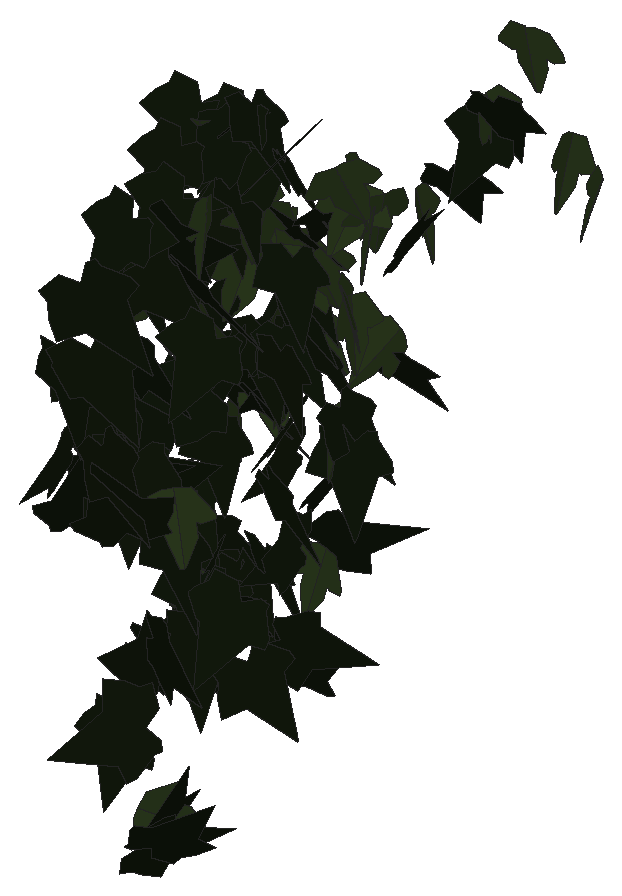
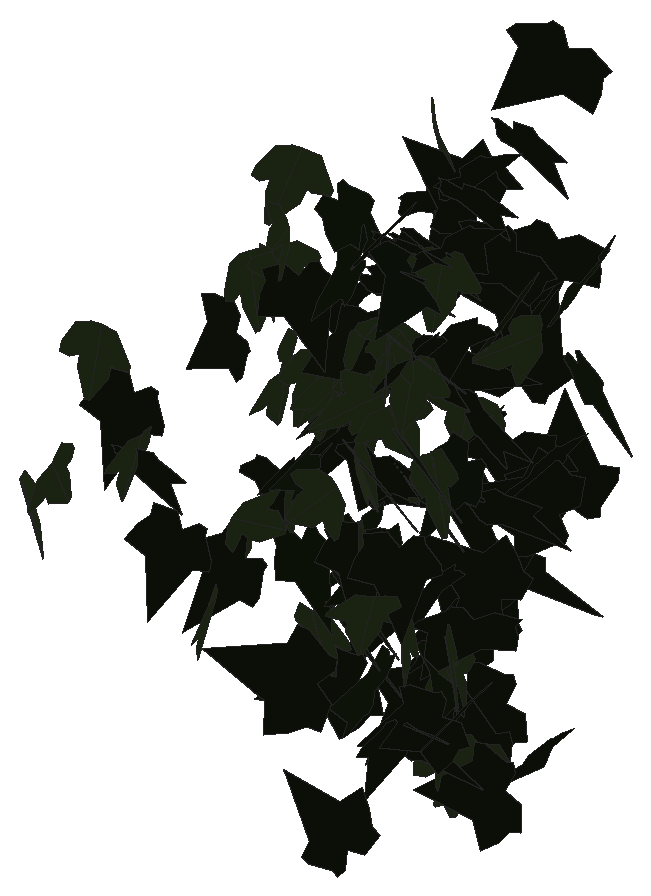
# SketchUp Ruby script. Lengths in inches.
U = 1.inch
M = Sketchup.active_model
def pt(a) = Geom::Point3d.new(a.map { |v| v * U })
def face(e, loops, mat)
  f = e.add_face(loops[0].map { |a| pt(a) })
  loops[1..].each { |l| e.add_face(l.map { |a| pt(a) }).erase! }
  f.material = f.back_material = mat if mat
  f
end
# faces: each face lists its corners as indices into pts; further lists are holes
def faces(e, pts, list, mat = nil) = list.each { |f| face(e, (f[0].is_a?(Array) ? f : [f]).map { |l| l.map { |i| pts[i] } }, mat) }
# xy, xz, yz: faces in a plane at the given z, y or x. An outline is a flat list of corners, or four numbers for a rectangle; further outlines are holes
def ring(l) = l.size == 4 ? [[l[0], l[1]], [l[2], l[1]], [l[2], l[3]], [l[0], l[3]]] : l.each_slice(2).to_a
def flat(e, list, mat, &to3) = list.each { |f| face(e, (f[0].is_a?(Array) ? f : [f]).map { |l| ring(l).map { |u, v| to3.(u, v) } }, mat) }
def xy(e, z, list, mat = nil) = flat(e, list, mat) { |x, y| [x, y, z] }
def xz(e, y, list, mat = nil) = flat(e, list, mat) { |x, z| [x, y, z] }
def yz(e, x, list, mat = nil) = flat(e, list, mat) { |y, z| [x, y, z] }
def lines(e, pts, list) = list.each { |a, b| e.add_line(pt(pts[a]), pt(pts[b])) }
# prism: a flat outline (further loops are holes) pulled along v
def prism(e, loops, v, mat = nil)
  f = face(e, loops, mat); d = Geom::Vector3d.new(v.map { |x| x * U })
  f.pushpull(f.normal.samedirection?(d) ? d.length : -d.length)
end
def box(e, o, s, mat = nil) = prism(e, [[o, [o[0] + s[0], o[1], o[2]], [o[0] + s[0], o[1] + s[1], o[2]], [o[0], o[1] + s[1], o[2]]]], [0, 0, s[2]], mat)
def at(x, y, z, deg = 0) = Geom::Transformation.translation(pt([x, y, z])) * Geom::Transformation.rotation(ORIGIN, Z_AXIS, deg.degrees)
def axes(o, x, y, z) = Geom::Transformation.new([*x, 0, *y, 0, *z, 0, *pt(o).to_a, 1])
def part(name) = M.definitions.add(name)
# library, detail: a bought-in or finely detailed component or shape, given as its bounding box
def library(name, o, s) = part(name).tap { |d| box(d.entities, o, s) }
def detail(e, o, s) = box(e.add_group.entities, o, s)
def put(e, d, t, mat = nil) = e.add_instance(d, t).tap { |i| i.material = mat if mat }
def group(e, t, mat = nil) = e.add_group.tap { |g| g.transformation = t; g.material = mat if mat }.entities
root = M.entities
M.materials.add("efeu1").color = [18, 25, 13]
M.materials.add("efeu2").color = [43, 57, 29]
c1 = part("ivyleaf_9")
p = [[1.54,2.16,1.25],[1.36,2.04,1.19],[-0.21,0.99,0.68],[-0.71,1.11,0.82],[-0.85,0.86,0.67],[-0.8,0.17,0.21],
  [-0.9,-0.01,0.1],[-0.67,-0.16,-0.02],[-0.08,-0.08,-0.05],[-0.03,-0.6,-0.4],[0.65,-0.88,-0.66],[0.83,-0.6,-0.49],
  [1.29,-0.42,-0.43],[1.8125,-0.07,-0.26],[1.21,0.44,0.15]]
faces(c1.entities,p,[[0,1,2,3,4,5,6,7,8,9,10,11,12,13,14]],"efeu1")
c2 = part("ivyleaf_10")
p = [[0,0.5,-0.03],[-0.0625,2.02,-0.43],[-0.19,2.01,-0.46],[-0.54,1.05,-0.29],[-0.52,0.625,-0.18],[-0.83,0.76,-0.28],
  [-1.16,0.64,-0.33],[-1.15,0.33,-0.24],[-0.77,-0.39,0.02],[-0.3,-0.51,0.16],[0.04,-0.48,0.23],[-0.02,2.01,-0.4375],
  [-0.06,2.01,-0.43],[0.04,-0.49,0.23],[0.67,-0.49,0.14],[1.38,0.36,-0.2],[1.375,0.51,-0.24],[0.81,0.65,-0.19],
  [0.62,0.59,-0.15],[0.6,1.09,-0.28],[0.5,1.23,-0.31]]
faces(c2.entities,p,[[0,1,2,3,4,5,6,7,8,9,10],[11,12,0,13,14,15,16,17,18,19,20]],"efeu2")
put(root,c1,axes([619.71,124.51,283.11],[0.14104,-1.19412,0.29819],[0.1203,-0.28533,-1.19952],[1.22489,0.16552,0.08347]))
put(root,c1,axes([620.89,120.86,290.27],[-1.22658,-0.3044,0.27362],[-0.25617,-0.10322,-1.26323],[0.31922,-1.25248,0.03761]))
put(root,c2,axes([621.07,124.15,293.12],[-1.02043,0.15526,0.7213],[-0.71477,0.09726,-1.03213],[-0.18297,-1.24583,0.00931]))
put(root,c1,axes([620.45,124.16,302.85],[-0.63355,-1.14175,0.20824],[-0.09383,-0.18608,-1.30572],[1.15678,-0.64041,0.00813]))
put(root,c1,axes([619.36,122.1,279.07],[0.35775,0.26821,-1.29353],[1.10185,0.67868,0.44547],[0.72874,-1.15784,-0.03852]))
put(root,c2,axes([620.8,124.01,301.91],[-1.19754,-0.39134,-0.00449],[0.00757,-0.00871,-1.25981],[0.39129,-1.19751,0.01063]))
put(root,c2,axes([620.59,126.33,287.7],[0.90865,-0.75502,-0.17753],[0.07219,0.35458,-1.13854],[0.77224,0.85523,0.31532]))
put(root,c1,axes([621.45,125.08,294.42],[-0.97791,0.66456,0.19935],[-0.14,0.14843,-1.18155],[-0.67954,-0.98693,-0.04346]))
put(root,c1,axes([620.97,126.21,290.59],[0.4329,1.00584,-0.46759],[-0.18238,-0.43056,-1.09504],[-1.09412,0.46975,-0.00247]))
put(root,c2,axes([621.11,123.04,285.32],[0.59435,-0.83326,-0.75214],[-0.36694,0.66008,-1.02124],[1.06084,0.69516,0.06815]))
put(root,c1,axes([620.08,124.93,283.17],[0.05345,0.10975,-1.2024],[0.74462,0.94445,0.1193],[0.95045,-0.74609,-0.02585]))
put(root,c2,axes([621.01,125.46,298],[-1.13515,-0.3909,-0.04214],[0.03774,0.01983,-1.20055],[0.39135,-1.13576,-0.00646]))
put(root,c1,axes([620.26,122.74,286.3],[-0.14041,-1.03973,-1.01108],[0.48333,0.92419,-1.0175],[1.36737,-0.43344,0.25583]))
put(root,c1,axes([619.99,121.53,286.98],[0.14228,-0.13325,1.28343],[1.21782,-0.41287,-0.17787],[0.42645,1.22351,0.07975]))
put(root,c1,axes([621.65,124.82,281.67],[-1.14568,-0.08665,0.29386],[-0.29432,-0.00458,-1.14883],[0.08508,-1.18276,-0.01708]))
put(root,c1,axes([621.73,125.75,299.33],[-1.15907,0.35504,0.07558],[-0.14039,-0.20526,-1.18885],[-0.33475,-1.14325,0.23692]))
put(root,c1,axes([620.82,122.49,292.72],[1.13415,0.1277,-0.38192],[-0.38987,0.06236,-1.13692],[-0.10084,1.1951,0.10014]))
put(root,c1,axes([620.88,118.46,290.43],[-0.25813,-1.36165,0.55677],[-0.07315,-0.5527,-1.3856],[1.46927,-0.26674,0.02883]))
put(root,c2,axes([620.85,127.98,289.04],[0.67829,0.94599,0.19596],[0.14933,0.1339,-1.16325],[-0.95447,0.69322,-0.04273]))
put(root,c1,axes([620.2,117.89,288.82],[0.62101,-0.04175,1.2435],[1.23146,0.21904,-0.60764],[-0.17763,1.37258,0.13479]))
put(root,c2,axes([620.89,118.57,296.3],[0.05214,-0.0986,-1.2203],[0.59241,1.07092,-0.06122],[1.0714,-0.58735,0.09323]))
put(root,c2,axes([621.16,137.3,292.93],[-0.48293,1.08305,-0.0953],[0.03791,-0.08744,-1.18584],[-1.08657,-0.48441,0.00098]))
put(root,c1,axes([620.91,125.72,298.5625],[0.14764,-1.20141,-0.09832],[-0.02428,0.09607,-1.21038],[1.20518,0.14911,-0.01234]))
put(root,c1,axes([620.99,124.7,288.24],[0.04342,-1.18127,-0.1517],[-0.02052,0.15104,-1.18197],[1.19079,0.04568,-0.01484]))
put(root,c1,axes([620.79,119.51,298.11],[0.74053,-1.03022,-0.2197],[-0.12507,0.18067,-1.26875],[1.04593,0.75101,0.00384]))
put(root,c1,axes([621.0625,115.95,288.1875],[1.10378,0.62926,0.69494],[-0.63864,-0.2812,1.26898],[0.68633,-1.27366,0.06318]))
put(root,c1,axes([621.13,123.48,298.47],[-0.35964,-1.19282,-0.28092],[0.0591,0.27555,-1.24566],[1.22403,-0.36378,-0.0224]))
put(root,c1,axes([621.57,124.08,301.63],[0.48511,1.03783,0.50874],[0.14861,0.49114,-1.14365],[-1.14622,0.50292,0.06703]))
put(root,c2,axes([621.91,121.93,279.83],[-1.13771,-0.48244,0.16954],[-0.14437,-0.09368,-1.23541],[0.49056,-1.14645,0.02961]))
put(root,c1,axes([622.25,113.72,292.47],[-0.98253,0.82327,-0.1504],[0.12281,-0.0876,-1.2818],[-0.82784,-0.99011,-0.01165]))
put(root,c1,axes([621.39,118.23,277.83],[-0.173,-1.2399,0.40661],[0.0437,-0.41544,-1.24824],[1.30414,-0.15056,0.09576]))
put(root,c1,axes([622.48,123.81,292.23],[-1.04024,0.59847,0.02572],[-0.02217,0.01304,-1.20011],[-0.59861,-1.04047,-0.00024]))
put(root,c2,axes([621.86,125.44,295.78],[0.67812,0.91424,-0.45354],[-0.28481,-0.35337,-1.13815],[-0.98,0.73531,0.01694]))
put(root,c1,axes([622.34,121.8,283.04],[-0.08767,0.80037,0.89248],[-0.18407,0.87527,-0.80302],[-1.18459,-0.19524,0.05873]))
put(root,c1,axes([622.45,123.66,302.21],[-1.22899,-0.03423,0.10312],[-0.10303,-0.00484,-1.22947],[0.03451,-1.2333,0.00196]))
put(root,c2,axes([621.87,125.89,298.55],[-0.77776,0.88381,-0.26604],[-0.01544,-0.36031,-1.15185],[-0.92285,-0.73883,0.24348]))
put(root,c1,axes([622.0625,124.875,302.81],[-1.08425,-0.51385,-0.31973],[0.41686,-0.15853,-1.15886],[0.43874,-1.11924,0.31093]))
put(root,c1,axes([623.17,119.01,292.53],[-0.72119,-0.09403,-1.15741],[-1.14799,-0.14736,0.72729],[-0.1748,1.35573,-0.00123]))
put(root,c1,axes([621.72,125.09,282.21],[0.1964,-1.04918,-0.76938],[-0.16739,0.75125,-1.06719],[1.29024,0.25717,-0.02134]))
put(root,c1,axes([622.27,120.64,303.1],[-1.11254,-0.43196,-0.34232],[0.37054,-0.01534,-1.1849],[0.40801,-1.16391,0.14266]))
put(root,c2,axes([621.75,125.72,299.09],[-1.02083,0.01451,-0.65115],[0.61566,-0.37352,-0.97352],[-0.21252,-1.15177,0.30751]))
put(root,c2,axes([622.19,121.76,282.96],[0.22086,1.06954,-0.4992],[-0.15707,-0.47671,-1.09086],[-1.16981,0.26594,0.05222]))
put(root,c1,axes([621.79,125.77,289.61],[1.12861,-0.38999,0.11606],[0.1102,-0.03645,-1.19408],[0.39168,1.13397,0.00153]))
put(root,c1,axes([622.73,126.01,290.17],[0.26275,1.17056,-0.10061],[-0.0087,-0.10115,-1.19961],[-1.17485,0.26254,-0.01361]))
put(root,c1,axes([623.44,125.21,293],[-0.78796,0.73862,0.52652],[-0.41896,0.32222,-1.07903],[-0.80452,-0.89122,0.04624]))
put(root,c1,axes([623.19,124.74,300.92],[-1.15389,-0.28579,0.27278],[-0.23947,-0.16383,-1.18464],[0.31423,-1.17432,0.09889]))
put(root,c1,axes([622.11,113.87,296.16],[0.38619,-1.27928,0.47772],[0.15322,-0.45273,-1.33621],[1.35694,0.41521,0.01492]))
put(root,c2,axes([623.0625,125.04,298.57],[-0.64427,-0.99951,0.20194],[-0.06467,-0.19835,-1.18801],[1.01766,-0.64539,0.05236]))
put(root,c1,axes([622.63,117.36,290.73],[-0.86915,-0.97202,-0.69466],[0.44139,0.53701,-1.30368],[1.1102,-0.97447,-0.02552]))
put(root,c2,axes([622.93,126.06,290.37],[0.63353,-0.8754,-0.53165],[-0.01623,0.61648,-1.03442],[1.02407,0.55133,0.31251]))
put(root,c2,axes([622.53,126.15,296.5],[0.06789,0.32976,1.1521],[0.29484,1.11388,-0.33619],[-1.16153,0.30202,-0.01799]))
put(root,c1,axes([622.46,124.3,300.18],[0.39553,-1.18119,0.1387],[0.03053,-0.13604,-1.24557],[1.18891,0.39646,-0.01416]))
put(root,c1,axes([622.74,122.15,282.02],[0.95512,0.70143,0.23417],[0.17258,0.16052,-1.18471],[-0.71907,0.97021,0.02671]))
put(root,c2,axes([622.98,125.95,293.5625],[0.58147,-0.9853,0.38409],[0.20769,-0.32339,-1.144],[1.03692,0.6173,0.01375]))
put(root,c1,axes([622.8,121.37,283.66],[-0.16151,-1.27801,0.00394],[-0.00142,-0.00379,-1.28818],[1.27802,-0.16151,-0.00094]))
put(root,c1,axes([622.54,124.99,303.16],[0.53288,-1.09982,-0.21322],[0.01137,0.24141,-1.2168],[1.12024,0.52071,0.11378]))
put(root,c1,axes([623.08,136.6875,295.22],[0.96369,0.62132,-0.34368],[-0.29163,-0.1819,-1.14661],[-0.64738,1.00684,0.00493]))
put(root,c1,axes([622.25,117.78,299.25],[0.13275,-0.51174,-1.39149],[0.96916,1.0872,-0.30737],[1.12199,-0.87856,0.43014]))
put(root,c1,axes([624.0625,125.6,287.87],[-1.04407,0.59078,-0.08696],[0.07461,-0.04473,-1.19962],[-0.59246,-1.04673,0.00218]))
put(root,c1,axes([623.06,124.96,293.2],[-0.669,-0.52372,-0.96245],[0.82525,0.50099,-0.84624],[0.7208,-1.05966,0.07559]))
put(root,c1,axes([623.97,115.41,302.71],[-1.25829,-0.21042,-0.3111],[0.30482,0.06335,-1.2757],[0.21943,-1.29462,-0.01186]))
put(root,c1,axes([623.94,118.64,302.28],[-0.71624,-0.97569,0.43488],[-0.20452,-0.38865,-1.20881],[1.04846,-0.74234,0.06129]))
put(root,c1,axes([624.34,125.2,289.69],[-0.75605,0.87844,-0.32614],[0.19144,-0.26542,-1.15868],[-0.91727,-0.77945,0.02699]))
put(root,c1,axes([623.1875,125.04,283.26],[0.78044,-1.0117,0.33632],[0.20451,-0.26701,-1.27774],[1.04634,0.80679,-0.00112]))
put(root,c2,axes([623.47,127.51,292.72],[-0.8731,0.14815,-0.79472],[0.76545,-0.22477,-0.88284],[-0.26004,-1.15904,0.06963]))
put(root,c1,axes([623.0625,126.83,277.48],[0.01946,-0.26493,1.2844],[1.11833,-0.66759,-0.15465],[0.68499,1.09744,0.21599]))
put(root,c1,axes([625.06,118.93,293.96],[-0.50475,-0.53842,-1.19678],[-0.78195,-0.90637,0.73756],[-1.05391,0.93035,0.02594]))
put(root,c1,axes([623.47,113.68,297.41],[-0.3999,-0.71245,-1.16865],[0.59825,1.00407,-0.81683],[1.23103,-0.71939,0.01732]))
put(root,c1,axes([623.21,125.57,298.21],[1.07144,-0.38469,0.4275],[0.43126,-0.06057,-1.13537],[0.38047,1.15198,0.08306]))
put(root,c1,axes([624.07,124.9,301.37],[1.05787,-0.51386,-0.29762],[-0.26183,0.1421,-1.176],[0.53298,1.08971,0.01301]))
put(root,c1,axes([624.0625,126.08,296.07],[0.55379,-1.04409,-0.22406],[-0.00137,0.2517,-1.17629],[1.06786,0.54179,0.11468]))
put(root,c1,axes([623.67,115.9375,296.53],[0.17162,0.07654,-1.2715],[1.20205,0.41479,0.18721],[0.42149,-1.21413,-0.0162]))
put(root,c1,axes([624.8,115.84,282.8],[-0.09999,-0.05994,1.23584],[-0.64275,-1.05693,-0.10327],[1.05725,-0.64823,0.0541]))
put(root,c1,axes([624.94,136.96,297.91],[-1.13051,-0.31041,-0.27835],[0.27005,0.0677,-1.17234],[0.31765,-1.16231,0.00605]))
put(root,c2,axes([624.375,116.37,275.78],[0.20212,0.50464,1.11578],[0.39776,1.0425,-0.54356],[-1.15819,0.44609,0.00805]))
put(root,c1,axes([624.38,124.65,293.84],[0.26473,-0.96776,-0.66949],[-0.01026,0.6843,-0.99322],[1.17672,0.22369,0.14196]))
put(root,c2,axes([624.77,137.18,298.56],[-0.12632,1.19336,0.10403],[-0.01308,0.10323,-1.20002],[-1.19781,-0.12698,0.00214]))
put(root,c1,axes([625.4375,124.09,302.96],[-0.73313,0.82699,-0.51134],[0.10561,-0.56889,-1.07148],[-0.96656,-0.68943,0.27077]))
put(root,c1,axes([623.98,118.9,298.78],[1.30129,-0.53558,0.38455],[0.35456,-0.14889,-1.4072],[0.55589,1.34873,-0.00264]))
put(root,c1,axes([625.74,123.75,284.99],[-1.0889,0.63883,0.13083],[-0.11082,0.06965,-1.26245],[-0.6426,-1.09451,-0.00398]))
put(root,c2,axes([624.84,125.43,295.92],[0.2776,1.16649,0.12122],[0.01229,0.12167,-1.19896],[-1.17271,0.2774,0.01613]))
put(root,c1,axes([624.46,124.92,295.57],[0.80442,-0.88299,-0.17271],[-0.0278,0.20718,-1.18866],[0.89929,0.79624,0.11775]))
put(root,c1,axes([624.04,117.94,300.65],[0.26796,-0.31854,1.34313],[1.13439,-0.72877,-0.39916],[0.78653,1.15961,0.1181]))
put(root,c1,axes([624.78,116.1,275.2],[0.39333,1.1447,0.66219],[-0.23359,-0.61986,1.21027],[1.30164,-0.45714,0.01709]))
put(root,c2,axes([625.13,125.7,296.8],[-0.831,-0.78669,-0.40615],[0.33594,0.2352,-1.1429],[0.81913,-0.89454,0.05668]))
put(root,c1,axes([624.93,118.55,283.14],[0.03198,-1.35517,-0.01433],[-0.00149,0.0143,-1.35555],[1.35525,0.03199,-0.00115]))
put(root,c1,axes([624.9,112.7,293.91],[0.75805,-1.11985,-0.5426],[-0.294,0.45619,-1.35225],[1.20915,0.81299,0.01138]))
put(root,c2,axes([625.59,129.67,291.7],[-0.34469,-0.48608,1.04457],[0.11332,-1.09933,-0.47417],[1.14654,-0.03748,0.3609]))
put(root,c1,axes([625.71,113.01,290.53],[0.99404,0.23425,1.01453],[-0.98966,-0.22337,1.02125],[0.3236,-1.40268,0.0068]))
put(root,c1,axes([625.31,130.2,290.42],[1.1579,0.32052,-0.06017],[-0.06725,0.01752,-1.20094],[-0.31911,1.15933,0.03478]))
put(root,c1,axes([626.78,112.68,282.13],[-1.30294,0.04477,0.61869],[-0.61789,0.03319,-1.30367],[-0.05467,-1.44199,-0.01079]))
put(root,c1,axes([625.21,122.81,288.09],[0.99009,-0.7996,-0.19163],[-0.13937,0.1324,-1.27256],[0.81035,0.99973,0.01527]))
put(root,c1,axes([625.14,125.86,292.92],[0.82821,-0.88045,0.09053],[0.09862,-0.03142,-1.20772],[0.87958,0.83255,0.05017]))
put(root,c1,axes([624.85,126.58,283.74],[0.7164,0.83411,-0.95031],[0.52065,0.80075,1.09534],[1.15228,-0.8804,0.0959]))
put(root,c1,axes([626.4,125.35,299.9375],[0.00377,1.13496,-0.42983],[-0.19325,-0.42379,-1.1207],[-1.19814,0.07193,0.1794]))
put(root,c1,axes([625.36,123.21,293.78],[0.43875,-1.10688,0.21512],[0.09772,-0.19263,-1.1905],[1.12335,0.44908,0.01955]))
put(root,c1,axes([625.98,135.875,299.6875],[1.04832,0.46198,-0.49603],[-0.43796,-0.23562,-1.14504],[-0.51736,1.13556,-0.03579]))
put(root,c1,axes([626.75,124.76,288.2],[-0.39085,1.1112,-0.27155],[0.05978,-0.26672,-1.17752],[-1.14234,-0.39415,0.03129]))
put(root,c1,axes([625.8,115.92,289.15],[0.37523,-1.33961,-0.14677],[-0.03558,0.14245,-1.39116],[1.34716,0.37689,0.00414]))
put(root,c2,axes([625.93,115.75,290.52],[1.10837,0.46078,0.33823],[0.32323,0.10335,-1.20002],[-0.47142,1.15421,-0.02758]))
put(root,c2,axes([625.99,117.53,302.89],[0.85375,-0.55107,0.72463],[0.58702,-0.42607,-1.01564],[0.69583,1.03559,-0.03226]))
put(root,c1,axes([626.05,123.05,298.33],[0.03765,-1.19958,-0.181],[0.04184,0.18226,-1.19925],[1.21244,0.03096,0.047]))
put(root,c2,axes([626.71,137.125,302.41],[-1.21064,-0.06486,-0.03905],[0.04542,-0.12161,-1.20604],[0.06057,-1.20515,0.1238]))
put(root,c2,axes([626.63,124,284.6],[1.17604,-0.24952,-0.06652],[-0.06751,0.00227,-1.20216],[0.24925,1.17792,-0.01177]))
put(root,c1,axes([626.41,113.25,276.4],[0.06388,0.78312,-1.06902],[0.10448,1.06395,0.78566],[1.32105,-0.12202,-0.01044]))
put(root,c1,axes([626.13,109.83,303],[-0.30101,-0.37439,-1.43914],[0.90048,1.12261,-0.48039],[1.18339,-0.94946,-0.00052]))
put(root,c1,axes([626.12,122.46,281.53],[0.34599,0.21406,-1.23678],[0.51304,1.14672,0.34199],[1.14553,-0.57823,0.22038]))
put(root,c1,axes([625.88,114.67,284.82],[0.47385,-0.1849,-1.36218],[1.37346,0.12404,0.46094],[0.05759,-1.4369,0.21508]))
put(root,c2,axes([627.32,125.48,300.52],[0.84906,0.7393,-0.47951],[-0.35601,-0.32132,-1.12579],[-0.80607,0.92065,-0.00786]))
put(root,c2,axes([627.27,124.9,296.36],[-0.78251,0.9289,0.0317],[-0.03025,0.01596,-1.2145],[-0.92894,-0.78299,0.01285]))
put(root,c2,axes([627.22,125.44,295.43],[-0.02573,1.19278,-0.26648],[0.02143,-0.26606,-1.19296],[-1.222,-0.02979,-0.01531]))
put(root,c2,axes([627,125,290.38],[0.02739,-0.62171,1.04311],[0.655,-0.87102,-0.53633],[1.02253,0.5746,0.31562]))
put(root,c2,axes([627.16,125.49,301.74],[-0.67297,0.61483,-0.8062],[0.50319,-0.63751,-0.90622],[-0.88021,-0.83452,0.09833]))
put(root,c2,axes([627.67,138.53,297.12],[0.01497,1.05734,-0.66458],[-0.08932,-0.66202,-1.05528],[-1.24565,0.06017,0.06769]))
put(root,c1,axes([627.36,124.6,291.36],[0.63761,-0.84412,-0.67888],[-0.23034,0.66408,-1.04206],[1.05847,0.653,0.18217]))
put(root,c2,axes([628.05,126.17,300.23],[-0.38848,-1.14887,0.01493],[-0.01934,-0.00922,-1.21267],[1.1488,-0.38865,-0.01536]))
put(root,c1,axes([627.51,118.51,282.67],[0.17654,-0.86219,-0.98097],[-0.12907,0.97353,-0.87888],[1.29962,0.21381,0.04596]))
put(root,c1,axes([628.13,115.47,298.78],[-0.70091,-1.03439,0.17022],[-0.10425,-0.13497,-1.24945],[1.04311,-0.70854,-0.01049]))
put(root,c1,axes([628.24,127,297.72],[0.25254,0.62101,1.0079],[0.22731,0.98596,-0.66445],[-1.16182,0.32789,0.08908]))
put(root,c2,axes([628.0625,125.36,299.76],[0.82676,-0.84888,0.3221],[0.28931,-0.16662,-1.18171],[0.86061,0.87151,0.08781]))
put(root,c1,axes([628.56,116.54,286.62],[-0.71547,-1.09559,0.17966],[-0.08324,-0.1602,-1.30839],[1.10709,-0.72008,0.01773]))
put(root,c1,axes([628.32,124.06,290.37],[-0.8248,-0.6044,-0.80135],[0.66929,0.44178,-1.02208],[0.74801,-1.06174,0.03089]))
put(root,c2,axes([628.57,122.95,303.07],[-0.85441,-0.7552,-0.45913],[0.36599,0.27895,-1.13991],[0.80448,-0.92898,0.03096]))
put(root,c2,axes([628.85,138.55,295.68],[0.70648,-1.01724,-0.1451],[-0.09868,0.10811,-1.23835],[1.02278,0.71308,-0.01925]))
put(root,c1,axes([628.41,111.48,277.9],[1.00708,0.87344,-0.11128],[0.07677,0.08132,1.33304],[0.87715,-1.00994,0.01109]))
